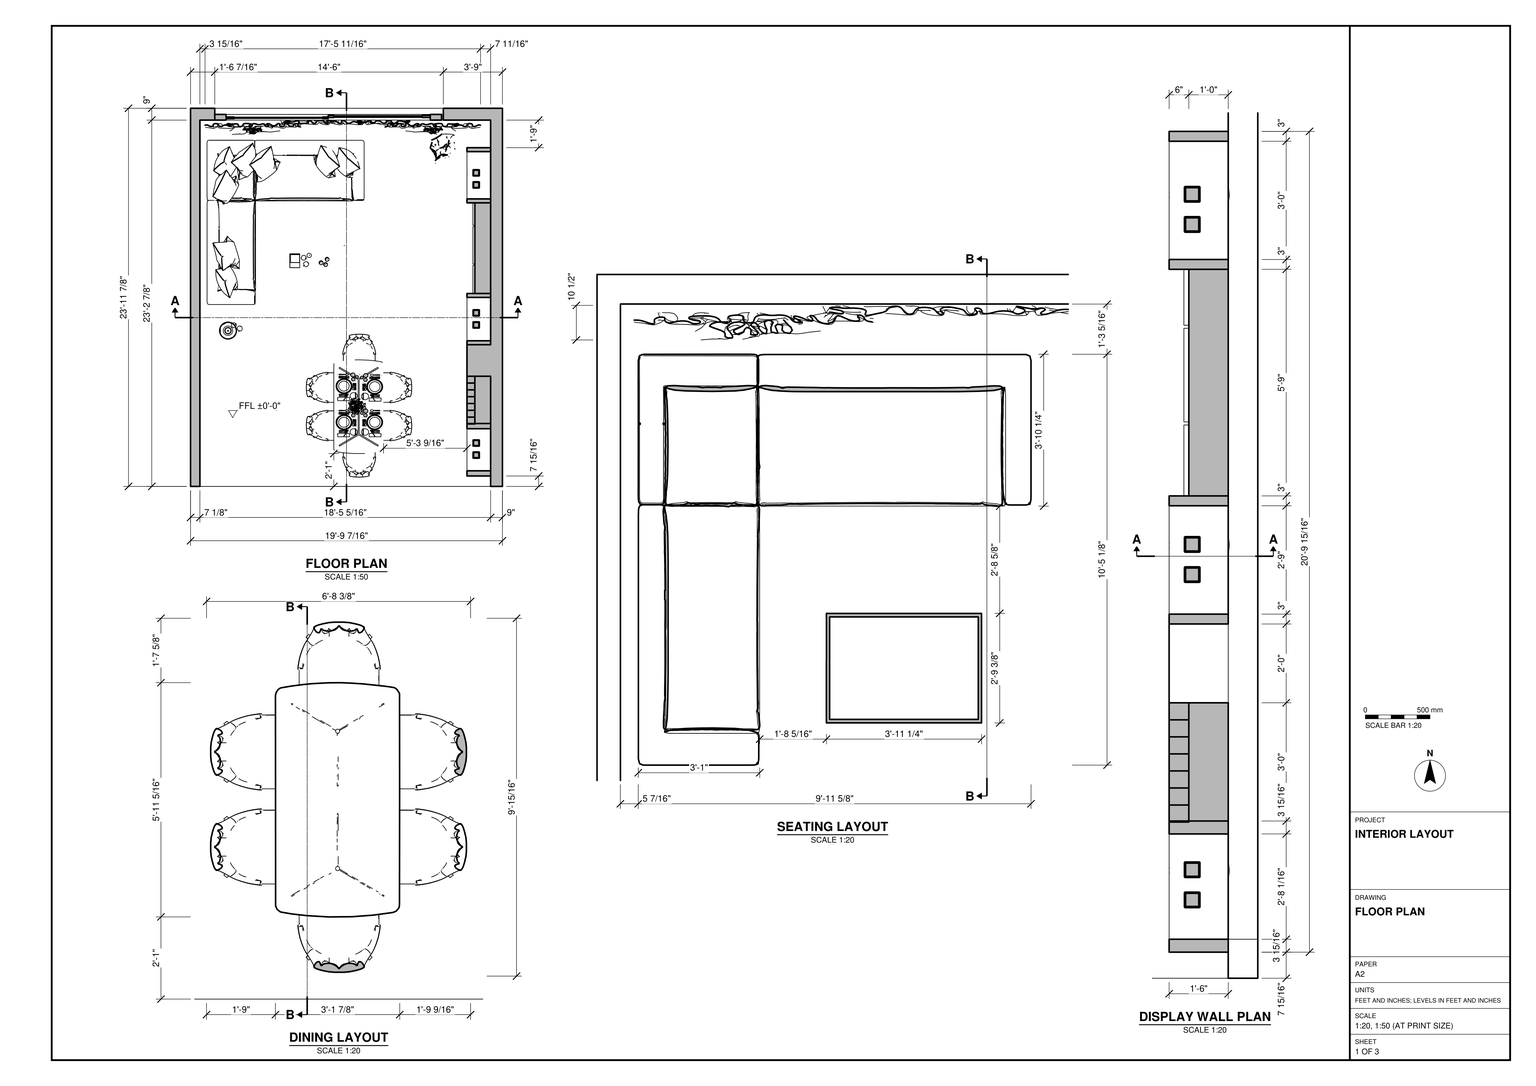
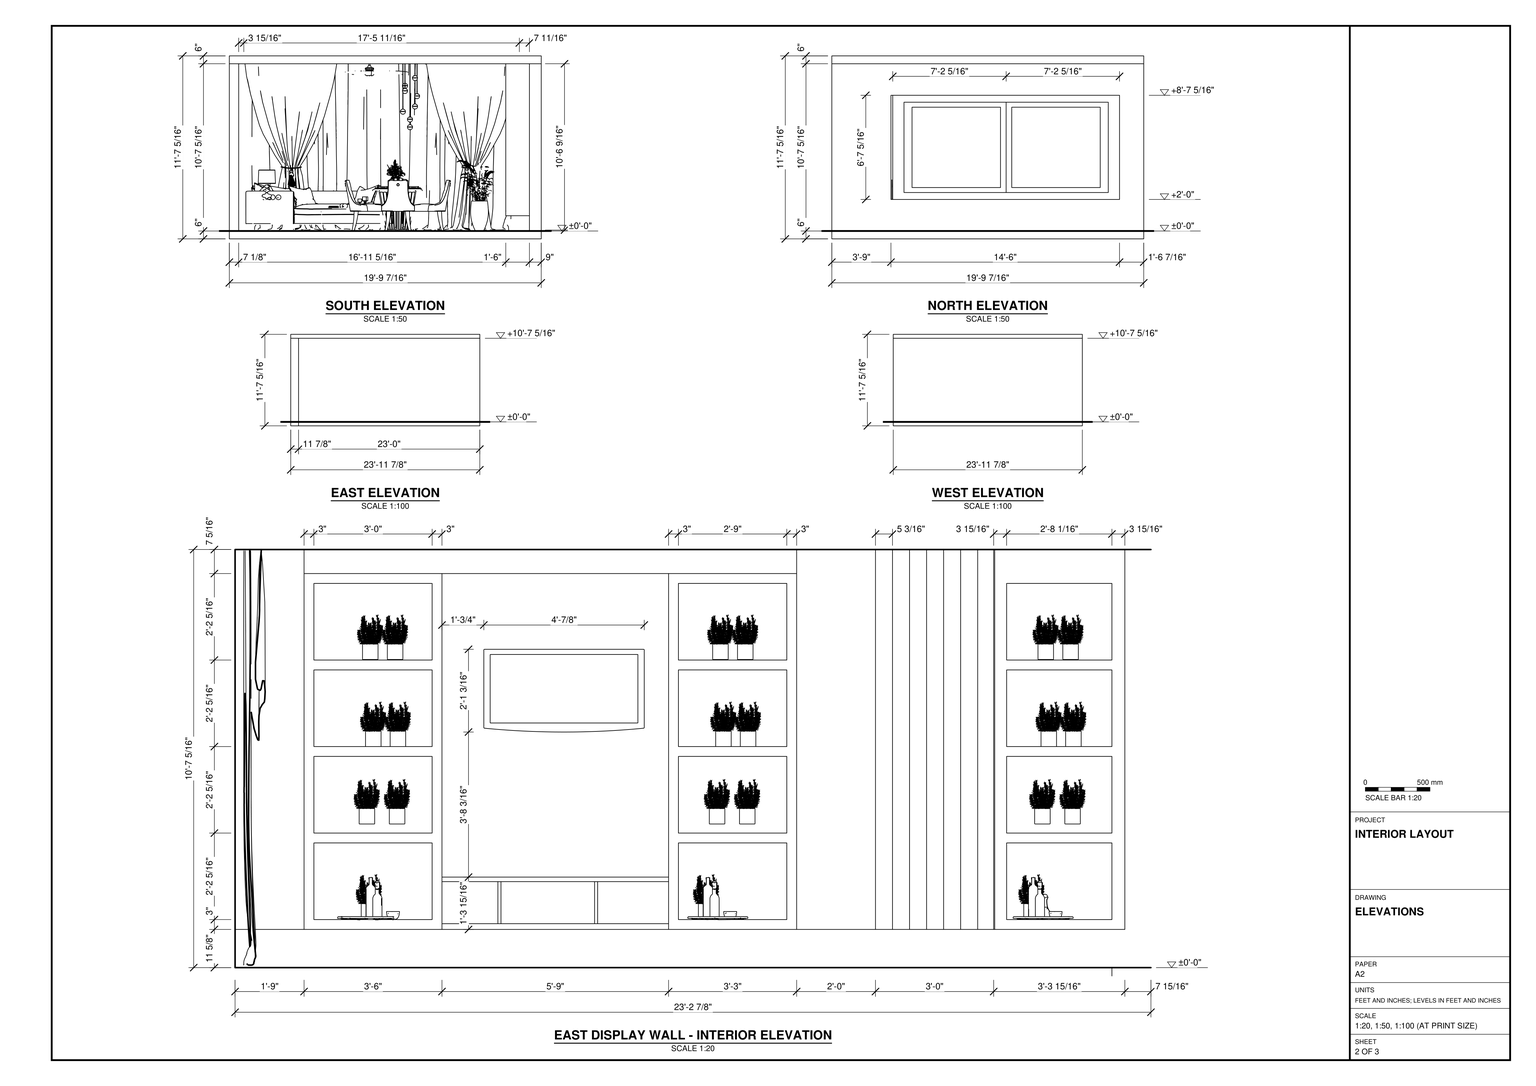
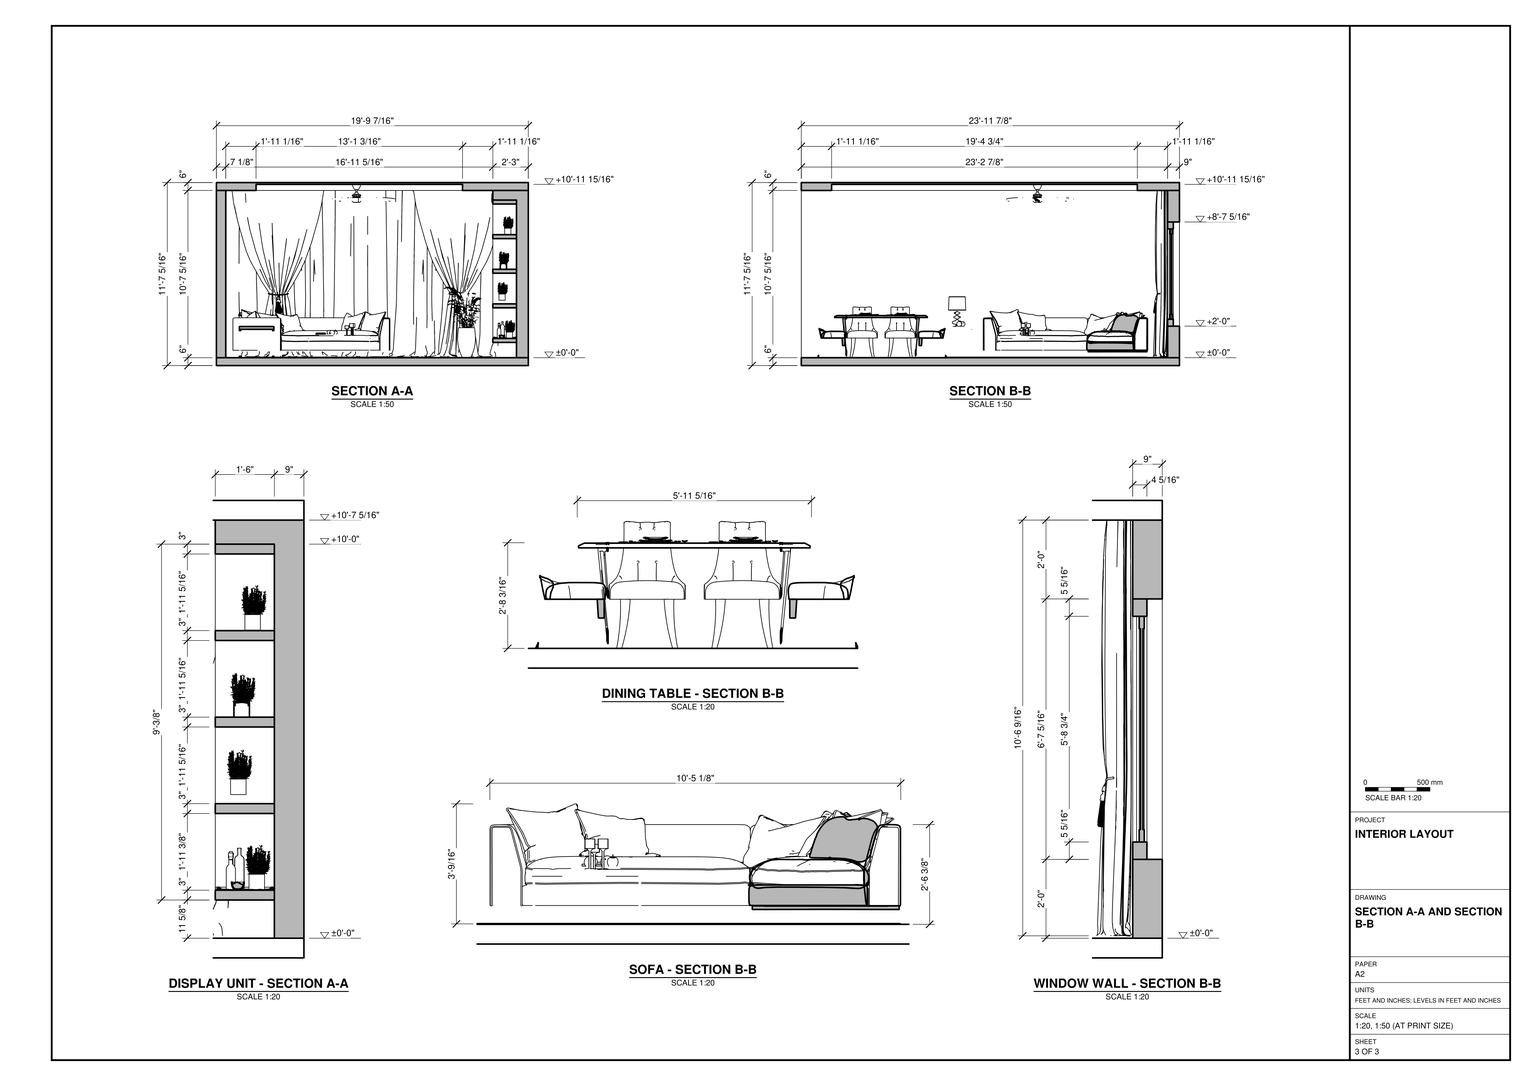
Build the furnished room shown in task_files/diagram_01.pdf. Work in feet and inches. Set the finished floor at ±0'-0" and orient the north window wall as shown in plan. The overall model measures 19'-9 7/16" east to west, 23'-11 7/8" north to south and 11'-7 5/16" high.

Model the floor slab, the west wall at 7 1/8" thick, and the north and east walls at 9" thick. Leave the south side open as drawn. Follow the sections for the slab thicknesses and recessed ceiling. Fit the wide, two-panel window into the north wall, with curtains on the room side. Place the L-shaped sofa in the northwest corner with the coffee table inside the L. In the southern part of the room, orient the dining table lengthwise north to south and arrange the chairs as shown in the dining layout.

Build the east display wall from its plan, interior elevation and section. Match the depth and spacing of the open shelf bays, the screen and low cabinet between the bays, and the vertically divided panel toward the dining end. Include the plants and shelf objects where shown. Decor and loose items may be any suitable library components.

Keep the shell elements and each furniture or joinery piece in separate groups or components, and use components for repeated parts. Save one SketchUp model as output_files/living_and_dining_room_with_built_in_display_shelving.skp.

# SketchUp Ruby script. Lengths in inches.
U = 1.inch
M = Sketchup.active_model
def pt(a) = Geom::Point3d.new(a.map { |v| v * U })
def face(e, loops, mat)
  f = e.add_face(loops[0].map { |a| pt(a) })
  loops[1..].each { |l| e.add_face(l.map { |a| pt(a) }).erase! }
  f.material = f.back_material = mat if mat
  f
end
# faces: each face lists its corners as indices into pts; further lists are holes
def faces(e, pts, list, mat = nil) = list.each { |f| face(e, (f[0].is_a?(Array) ? f : [f]).map { |l| l.map { |i| pts[i] } }, mat) }
# xy, xz, yz: faces in a plane at the given z, y or x. An outline is a flat list of corners, or four numbers for a rectangle; further outlines are holes
def ring(l) = l.size == 4 ? [[l[0], l[1]], [l[2], l[1]], [l[2], l[3]], [l[0], l[3]]] : l.each_slice(2).to_a
def flat(e, list, mat, &to3) = list.each { |f| face(e, (f[0].is_a?(Array) ? f : [f]).map { |l| ring(l).map { |u, v| to3.(u, v) } }, mat) }
def xy(e, z, list, mat = nil) = flat(e, list, mat) { |x, y| [x, y, z] }
def xz(e, y, list, mat = nil) = flat(e, list, mat) { |x, z| [x, y, z] }
def yz(e, x, list, mat = nil) = flat(e, list, mat) { |y, z| [x, y, z] }
def lines(e, pts, list) = list.each { |a, b| e.add_line(pt(pts[a]), pt(pts[b])) }
# prism: a flat outline (further loops are holes) pulled along v
def prism(e, loops, v, mat = nil)
  f = face(e, loops, mat); d = Geom::Vector3d.new(v.map { |x| x * U })
  f.pushpull(f.normal.samedirection?(d) ? d.length : -d.length)
end
def box(e, o, s, mat = nil) = prism(e, [[o, [o[0] + s[0], o[1], o[2]], [o[0] + s[0], o[1] + s[1], o[2]], [o[0], o[1] + s[1], o[2]]]], [0, 0, s[2]], mat)
def at(x, y, z, deg = 0) = Geom::Transformation.translation(pt([x, y, z])) * Geom::Transformation.rotation(ORIGIN, Z_AXIS, deg.degrees)
def axes(o, x, y, z) = Geom::Transformation.new([*x, 0, *y, 0, *z, 0, *pt(o).to_a, 1])
def part(name) = M.definitions.add(name)
# library, detail: a bought-in or finely detailed component or shape, given as its bounding box
def library(name, o, s) = part(name).tap { |d| box(d.entities, o, s) }
def detail(e, o, s) = box(e.add_group.entities, o, s)
def put(e, d, t, mat = nil) = e.add_instance(d, t).tap { |i| i.material = mat if mat }
def group(e, t, mat = nil) = e.add_group.tap { |g| g.transformation = t; g.material = mat if mat }.entities
root = M.entities
M.materials.add("Decor - Oil Bottle - Label").color = [52, 51, 50]
M.materials.add("Decor - Oil Bottles - Black Glass").color = [0, 0, 0]
M.materials["Decor - Oil Bottles - Black Glass"].alpha = 0.45
M.materials.add("[Carrera Marble]").color = [207, 207, 207]
M.materials.add("[Color D02]").color = [255, 241, 201]
M.materials.add("[Stone Brushed Khaki]").color = [226, 197, 133]
M.materials.add("[Translucent_Glass_Safety]").color = [204, 235, 244]
M.materials["[Translucent_Glass_Safety]"].alpha = 0.5
M.materials.add("[Translucent_Glass_Sky_Reflection]").color = [125, 138, 183]
M.materials["[Translucent_Glass_Sky_Reflection]"].alpha = 0.52
M.materials.add("[Wood Veneer 01]").color = [120, 70, 37]
c1 = library("Group14",[-64.97,9.24,0.31],[138.52,9.93,292.57])
c2 = library("Group16",[86.37,-10.76,76.46],[21.79,14.87,35.97])
c3 = library("Group22",[48.82,-10.91,0.23],[97.72,18.57,293.12])
c4 = library("Group24",[44.03,2.01,0.26],[103.73,11,292.35])
c5 = library("Group27",[-106.21,-10.76,76.46],[21.8,14.87,35.97])
c6 = library("Group35",[-145.81,2.01,0.26],[103.73,11,292.35])
c7 = library("Group33",[-144.59,-10.91,0.23],[97.72,18.57,293.12])
c8 = part("rem")
g1 = group(c8.entities,at(-145.81,-10.91,0.23))
put(g1,c1,at(145.81,10.91,-0.23))
put(g1,c2,at(145.81,10.91,-0.23))
put(g1,c3,at(145.81,10.91,-0.23))
put(g1,c4,at(145.81,10.91,-0.23))
put(g1,c5,at(145.81,10.91,-0.23))
put(g1,c6,at(145.81,10.91,-0.23))
put(g1,c7,at(145.81,10.91,-0.23))
c9 = part("Sliding window")
xy(c9.entities,0,[[0,0,4.33,55.51]])
xy(c9.entities,2.76,[[0,2.76,2,27.76],[3.15,2.76,4.33,27.76],[0,27.76,0.82,52.76],[0.82,27.76,2.36,52.76],[2.36,27.76,4.33,52.76]])
xy(c9.entities,4.72,[[2,4.72,2.4,26.38],[2.76,4.72,3.15,26.38],[0.82,29.13,1.22,50.79],[1.97,29.13,2.36,50.79]])
xy(c9.entities,36.61,[[2,4.72,2.4,26.38],[2.76,4.72,3.15,26.38],[0.82,29.13,1.22,50.79],[1.97,29.13,2.36,50.79]])
xy(c9.entities,38.58,[[0,2.76,2,27.76],[3.15,2.76,4.33,27.76],[0,27.76,0.82,52.76],[0.82,27.76,2.36,52.76],[2.36,27.76,4.33,52.76]])
xy(c9.entities,41.34,[[0,0,4.33,55.51]])
xz(c9.entities,0,[[0,0,4.33,41.34]])
xz(c9.entities,2.76,[[0,2.76,2,38.58],[3.15,2.76,4.33,38.58]])
xz(c9.entities,4.72,[[2,4.72,2.4,36.61],[2.76,4.72,3.15,36.61]])
xz(c9.entities,26.38,[[2,4.72,2.4,36.61],[2.76,4.72,3.15,36.61]])
xz(c9.entities,27.76,[[0.82,2.76,2,38.58],[2,2.76,2.36,38.58],[2.36,2.76,3.15,38.58]])
xz(c9.entities,29.13,[[0.82,4.72,1.22,36.61],[1.97,4.72,2.36,36.61]])
xz(c9.entities,50.79,[[0.82,4.72,1.22,36.61],[1.97,4.72,2.36,36.61]])
xz(c9.entities,52.76,[[0,2.76,0.82,38.58],[0.82,2.76,2.36,38.58],[2.36,2.76,4.33,38.58]])
xz(c9.entities,55.51,[[0,0,4.33,41.34]])
yz(c9.entities,0,[[[0,0,55.51,41.34],[2.76,2.76,52.76,38.58]]])
yz(c9.entities,0.82,[[[27.76,2.76,52.76,38.58],[29.13,4.72,50.79,36.61]]])
yz(c9.entities,1.22,[[29.13,4.72,50.79,36.61]],"[Translucent_Glass_Sky_Reflection]")
yz(c9.entities,1.97,[[29.13,4.72,50.79,36.61]],"[Translucent_Glass_Sky_Reflection]")
yz(c9.entities,2,[[[2.76,2.76,27.76,38.58],[4.72,4.72,26.38,36.61]]])
yz(c9.entities,2.36,[[[27.76,2.76,52.76,38.58],[29.13,4.72,50.79,36.61]]])
yz(c9.entities,2.4,[[4.72,4.72,26.38,36.61]],"[Translucent_Glass_Safety]")
yz(c9.entities,2.76,[[4.72,4.72,26.38,36.61]],"[Translucent_Glass_Safety]")
yz(c9.entities,3.15,[[[2.76,2.76,27.76,38.58],[4.72,4.72,26.38,36.61]]])
yz(c9.entities,4.33,[[[0,0,55.51,41.34],[2.76,2.76,52.76,38.58]]])
c10 = library("dinning+table+2",[29.07,47.92,0],[99.06,67.68,49.4])
c11 = library("Cluster pendant light",[0,0,0],[15.54,15.54,54.85])
c12 = library("Untitled",[82.71,28.87,-11.8125],[39.77,1.97,25.2])
c13 = library("Avation+Styled+Ceiling+Fan_JSB",[-19.77,-29.63,-13.8125],[51.59,58.16,13.8125])
c14 = library("Group3\#3",[-238.15,54.18,0],[46.4,43.96,56.68])
c15 = library("迷迭香盆栽   Potted rosemary    盆栽 Potted plants     迷迭香   Rosema",[-0.43,-2,0.01],[7.68,8.25,13.59])
c16 = library("Tepsi",[27.43,-114.7,10.73],[90.81,90.81,4.36])
c17 = library("Utensílios de cozinha - Galheteiro ",[91.875,-459.8125,1.36],[84.84,84.82,188.36])
c18 = part("Group\#1")
xy(c18.entities,115.6875,[[0,0,6,5.1875]])
xz(c18.entities,0,[[0,0,6,115.6875]])
yz(c18.entities,0,[[0,0,5.1875,115.6875]])
c19 = library("Group\#11",[0,0,0],[145.32,155.63,46.53])
c20 = library("Group325\#1",[30.57,-11.72,-14.39],[18.62,18.62,11.32])
c21 = library("Group318\#2",[50.77,-2.74,-14.76],[26.73,29.52,13.62])
c22 = library("Group\#44",[-0.82,-0.34,0],[4.09,3.62,11.67])
c23 = library("olive_Defintion19",[-63.02,-346.37,-115.47],[230.93,1000,230.94])
c24 = part("olive_Defintion")
p = [[49.84,-436.47,-188.95],[50.23,563.53,-187],[87.34,563.53,-190.7],[87.34,-436.47,-192.68],[124.45,563.53,-187],[124.84,-436.47,-188.95],
  [14.53,563.53,-176.21],[13.77,-436.47,-178.05],[160.15,563.53,-176.21],[160.91,-436.47,-178.05],[-19.44,-436.47,-160.25],[-18.34,563.53,-158.6],
  [193.02,563.53,-158.6],[194.12,-436.47,-160.25],[-45.45,563.53,-137.57],[-46.84,-436.47,-139],[220.13,563.53,-137.57],[221.52,-436.47,-139],
  [-65.45,-436.47,-117.73],[-63.87,563.53,-116.52],[238.55,563.53,-116.52],[240.13,-436.47,-117.73],[-77.94,563.53,-95.46],[-79.67,-436.47,-96.45],
  [252.625,563.53,-95.46],[254.35,-436.47,-96.45],[-65.45,-436.47,117.65],[-63.87,563.53,116.4375],[-77.94,563.53,95.375],[-79.67,-436.47,96.37],
  [252.625,563.53,95.375],[238.55,563.53,116.4375],[240.13,-436.47,117.65],[254.35,-436.47,96.37],[-45.45,563.53,137.49],[-46.84,-436.47,138.92],
  [220.13,563.53,137.49],[221.52,-436.47,138.92],[-19.44,-436.47,160.17],[-18.34,563.53,158.52],[193.02,563.53,158.52],[194.12,-436.47,160.17],
  [14.53,563.53,176.13],[13.77,-436.47,177.96],[160.15,563.53,176.13],[160.91,-436.47,177.96],[49.84,-436.47,188.87],[50.23,563.53,186.92],
  [124.45,563.53,186.92],[124.84,-436.47,188.87],[87.34,563.53,190.61],[87.34,-436.47,192.6]]
faces(c24.entities,p,[[0,1,2,3],[2,4,5,3],[6,1,0,7],[5,4,8,9],[10,11,6,7],[8,12,13,9],[14,11,10,15],[13,12,16,17],
  [18,19,14,15],[16,20,21,17],[22,19,18,23],[21,20,24,25],[26,27,28,29],[30,31,32,33],[34,27,26,35],[32,31,36,37],
  [38,39,34,35],[36,40,41,37],[42,39,38,43],[41,40,44,45],[46,47,42,43],[44,48,49,45],[50,47,46,51],[49,48,50,51]],"Decor - Oil Bottle - Label")
c25 = part("Group32\#1")
put(c25.entities,c23,axes([15235.87,28195.44,20659.33],[-10.1187,-7.58183,0],[0,0,12.64406],[-7.58183,10.1187,0]),"Decor - Oil Bottles - Black Glass")
put(c25.entities,c24,axes([15235.87,28195.44,20659.33],[-6.07632,-4.55292,0],[0,0,7.59281],[-4.55292,6.07632,0]),"Decor - Oil Bottle - Label")
c26 = part("Group31\#1")
put(c26.entities,c25,at(0,0,0))
xy(root,-6,[[0,0,237.4375,11.875],[0,11.875,237.4375,287.875]])
xy(root,0,[[0,0,7.125,11.875],[7.125,0,228.4375,278.875],[228.4375,0,237.4375,11.875],[0,11.875,7.125,11.875,7.125,278.875,228.4375,278.875,228.4375,11.875,237.4375,11.875,237.4375,287.875,0,287.875]])
xy(root,11.625,[[210.4375,7.9375,228.4375,11.875],[210.4375,11.875,228.4375,47.875],[216.4375,47.875,228.4375,83.875],[210.4375,78.6875,216.4375,83.875],[210.4375,83.875,228.4375,107.875],
  [210.4375,107.875,228.4375,146.875],[217.6875,146.875,228.4375,215.875],[210.4375,215.875,228.4375,257.875]])
xy(root,13.375,[[214.9375,146.875,216.4375,168.47],[216.4375,146.875,216.4375,198.85,214.9375,198.85,214.9375,215.875,217.6875,215.875,217.6875,146.875],[214.9375,169.41,216.4375,197.91]])
xy(root,14.625,[[210.4375,11.875,228.4375,43.9375],[210.4375,110.875,228.4375,143.875],[210.4375,218.875,228.4375,254.875]],"[Wood Veneer 01]")
xy(root,24,[[18.4375,278.875,192.4375,287.875]])
xy(root,26.1875,[[214.9375,146.875,216.4375,168.47],[216.4375,146.875,217.6875,146.875,217.6875,215.875,214.9375,215.875,214.9375,198.85,216.4375,198.85],[214.9375,169.41,216.4375,197.91]],"[Stone Brushed Khaki]")
xy(root,27.5625,[[216.4375,146.875,217.6875,215.875]])
xy(root,37.97,[[210.4375,11.875,228.4375,43.9375],[210.4375,110.875,228.4375,143.875],[210.4375,218.875,228.4375,254.875]])
xy(root,40.97,[[210.4375,11.875,228.4375,43.9375],[210.4375,110.875,228.4375,143.875],[210.4375,218.875,228.4375,254.875]],"[Wood Veneer 01]")
xy(root,64.3125,[[210.4375,11.875,228.4375,43.9375],[210.4375,110.875,228.4375,143.875],[210.4375,218.875,228.4375,254.875]])
xy(root,67.3125,[[210.4375,11.875,228.4375,43.9375],[210.4375,110.875,228.4375,143.875],[210.4375,218.875,228.4375,254.875]],"[Wood Veneer 01]")
xy(root,90.66,[[210.4375,11.875,228.4375,43.9375],[210.4375,110.875,228.4375,143.875],[210.4375,218.875,228.4375,254.875]])
xy(root,93.66,[[210.4375,11.875,228.4375,43.9375],[210.4375,110.875,228.4375,143.875],[210.4375,218.875,228.4375,254.875]],"[Wood Veneer 01]")
xy(root,103.3125,[[18.4375,278.875,192.4375,287.875]])
xy(root,117,[[210.4375,11.875,228.4375,43.9375],[210.4375,110.875,228.4375,143.875],[210.4375,218.875,228.4375,254.875]])
xy(root,120,[[210.4375,107.875,228.4375,146.875],[210.4375,146.875,216.4375,215.875],[216.4375,146.875,228.4375,215.875],[210.4375,215.875,228.4375,257.875]])
xy(root,127.3125,[[[7.125,0,7.125,278.875,228.4375,278.875,228.4375,257.875,210.4375,257.875,210.4375,83.875,216.4375,83.875,216.4375,47.875,210.4375,47.875,210.4375,7.9375,228.4375,7.9375,228.4375,0],[30.2,23.07,187.37,255.8]],[210.4375,7.9375,210.4375,47.875,216.4375,47.875,216.4375,83.875,228.4375,83.875,228.4375,7.9375]])
xy(root,127.3125,[[0,0,0,287.875,237.4375,287.875,237.4375,0,228.4375,0,228.4375,83.875,210.4375,83.875,210.4375,257.875,228.4375,257.875,228.4375,278.875,7.125,278.875,7.125,0],[210.4375,7.9375,228.4375,47.875],[216.4375,47.875,228.4375,83.875]],"[Wood Veneer 01]")
xy(root,131.9375,[[30.2,23.07,187.37,255.8]])
xy(root,133.3125,[[0,0,237.4375,287.875]])
xz(root,0,[[0,-6,237.4375,0],[0,0,7.125,127.3125],[228.4375,0,237.4375,127.3125],[0,127.3125,237.4375,133.3125]])
xz(root,7.9375,[[210.4375,11.625,228.4375,127.3125]],"[Wood Veneer 01]")
xz(root,11.875,[[210.4375,14.625,228.4375,37.97],[210.4375,40.97,228.4375,64.3125],[210.4375,67.3125,228.4375,90.66],[210.4375,93.66,228.4375,117]],"[Wood Veneer 01]")
xz(root,23.07,[[30.2,127.3125,187.37,131.9375]])
xz(root,43.9375,[[210.4375,14.625,228.4375,37.97],[210.4375,40.97,228.4375,64.3125],[210.4375,67.3125,228.4375,90.66],[210.4375,93.66,228.4375,117]],"[Wood Veneer 01]")
xz(root,47.875,[[210.4375,11.625,216.4375,127.3125],[216.4375,11.625,228.4375,127.3125]])
xz(root,83.875,[[210.4375,11.625,216.4375,127.3125],[216.4375,11.625,228.4375,127.3125]])
xz(root,107.875,[[210.4375,11.625,228.4375,120]])
xz(root,110.875,[[210.4375,14.625,228.4375,37.97],[210.4375,40.97,228.4375,64.3125],[210.4375,67.3125,228.4375,90.66],[210.4375,93.66,228.4375,117]],"[Wood Veneer 01]")
xz(root,143.875,[[210.4375,14.625,228.4375,37.97],[210.4375,40.97,228.4375,64.3125],[210.4375,67.3125,228.4375,90.66],[210.4375,93.66,228.4375,117]],"[Wood Veneer 01]")
xz(root,146.875,[[217.6875,11.625,217.6875,13.375,216.4375,13.375,216.4375,26.1875,217.6875,26.1875,217.6875,27.5625,216.4375,27.5625,216.4375,120,228.4375,120,228.4375,11.625],[214.9375,13.375,216.4375,26.1875]])
xz(root,146.875,[[210.4375,11.625,210.4375,120,216.4375,120,216.4375,27.5625,217.6875,27.5625,217.6875,26.1875,214.9375,26.1875,214.9375,13.375,217.6875,13.375,217.6875,11.625]],"[Wood Veneer 01]")
xz(root,168.47,[[214.9375,13.375,216.4375,26.1875]])
xz(root,169.41,[[214.9375,13.375,216.4375,26.1875]])
xz(root,197.91,[[214.9375,13.375,216.4375,26.1875]])
xz(root,198.85,[[214.9375,13.375,216.4375,26.1875]],"[Stone Brushed Khaki]")
xz(root,215.875,[[217.6875,11.625,228.4375,11.625,228.4375,120,216.4375,120,216.4375,27.5625,217.6875,27.5625,217.6875,26.1875,214.9375,26.1875,214.9375,13.375,217.6875,13.375]])
xz(root,215.875,[[210.4375,11.625,217.6875,11.625,217.6875,13.375,214.9375,13.375,214.9375,26.1875,217.6875,26.1875,217.6875,27.5625,216.4375,27.5625,216.4375,120,210.4375,120]],"[Wood Veneer 01]")
xz(root,218.875,[[210.4375,14.625,228.4375,37.97],[210.4375,40.97,228.4375,64.3125],[210.4375,67.3125,228.4375,90.66],[210.4375,93.66,228.4375,117]])
xz(root,254.875,[[210.4375,14.625,228.4375,37.97],[210.4375,40.97,228.4375,64.3125],[210.4375,67.3125,228.4375,90.66],[210.4375,93.66,228.4375,117]],"[Wood Veneer 01]")
xz(root,255.8,[[30.2,127.3125,187.37,131.9375]])
xz(root,257.875,[[210.4375,120,228.4375,127.3125]])
xz(root,257.875,[[210.4375,11.625,228.4375,120]],"[Wood Veneer 01]")
xz(root,278.875,[[[7.125,0,228.4375,127.3125],[18.4375,24,192.4375,103.3125]]],"[Color D02]")
xz(root,287.875,[[0,-6,237.4375,0],[[0,0,237.4375,127.3125],[18.4375,24,192.4375,103.3125]],[0,127.3125,237.4375,133.3125]])
yz(root,0,[[0,-6,287.875,0],[0,0,287.875,127.3125],[0,127.3125,287.875,133.3125]])
yz(root,7.125,[[0,0,278.875,127.3125]],"[Color D02]")
yz(root,18.4375,[[278.875,24,287.875,103.3125]])
yz(root,30.2,[[23.07,127.3125,255.8,131.9375]])
yz(root,187.37,[[23.07,127.3125,70.95,131.9375],[70.95,127.3125,107.875,131.9375],[107.875,127.3125,255.8,131.9375]])
yz(root,192.4375,[[278.875,24,287.875,103.3125]])
yz(root,210.4375,[[83.875,11.625,107.875,127.3125]],"[Color D02]")
yz(root,210.4375,[[[7.9375,11.625,47.875,127.3125],[11.875,14.625,43.9375,37.97],[11.875,67.3125,43.9375,90.66],[11.875,93.66,43.9375,117],[11.875,40.97,43.9375,64.3125]],[[107.875,11.625,146.875,120],[110.875,93.66,143.875,117],[110.875,67.3125,143.875,90.66],[110.875,14.625,143.875,37.97],[110.875,40.97,143.875,64.3125]],[[215.875,11.625,257.875,120],[218.875,93.66,254.875,117],[218.875,67.3125,254.875,90.66],[218.875,14.625,254.875,37.97],[218.875,40.97,254.875,64.3125]],[107.875,120,257.875,127.3125]],"[Wood Veneer 01]")
yz(root,214.9375,[[146.875,13.375,168.47,26.1875],[169.41,13.375,197.91,26.1875],[198.85,13.375,215.875,26.1875]],"[Stone Brushed Khaki]")
yz(root,216.4375,[[47.875,11.625,78.6875,127.3125],[78.6875,11.625,83.875,127.3125],[146.875,13.375,168.47,26.1875],[169.41,13.375,197.91,26.1875],[197.91,13.375,198.85,26.1875]])
yz(root,216.4375,[[146.875,27.5625,215.875,120]],"[Carrera Marble]")
yz(root,216.4375,[[168.47,13.375,169.41,26.1875]],"[Stone Brushed Khaki]")
yz(root,217.6875,[[146.875,11.625,215.875,13.375]])
yz(root,217.6875,[[146.875,26.1875,215.875,27.5625]],"[Stone Brushed Khaki]")
yz(root,228.4375,[[[7.9375,11.625,47.875,127.3125],[11.875,14.625,43.9375,37.97],[11.875,93.66,43.9375,117],[11.875,67.3125,43.9375,90.66],[11.875,40.97,43.9375,64.3125]],[47.875,11.625,83.875,127.3125],[[107.875,11.625,146.875,120],[110.875,93.66,143.875,117],[110.875,67.3125,143.875,90.66],[110.875,14.625,143.875,37.97],[110.875,40.97,143.875,64.3125]],[146.875,11.625,215.875,120],[[215.875,11.625,257.875,120],[218.875,93.66,254.875,117],[218.875,67.3125,254.875,90.66],[218.875,14.625,254.875,37.97],[218.875,40.97,254.875,64.3125]]])
yz(root,228.4375,[[0,0,0,127.3125,7.9375,127.3125,7.9375,11.625,278.875,11.625,278.875,0],[257.875,11.625,278.875,127.3125]],"[Color D02]")
yz(root,228.4375,[[11.875,14.625,43.9375,37.97],[110.875,14.625,143.875,37.97],[218.875,14.625,254.875,37.97],[11.875,40.97,43.9375,64.3125],[110.875,40.97,143.875,64.3125],
  [218.875,40.97,254.875,64.3125],[11.875,67.3125,43.9375,90.66],[110.875,67.3125,143.875,90.66],[218.875,67.3125,254.875,90.66],[11.875,93.66,43.9375,117],
  [110.875,93.66,143.875,117],[218.875,93.66,254.875,117]],"[Wood Veneer 01]")
yz(root,237.4375,[[0,-6,11.875,0],[11.875,-6,287.875,0],[0,0,11.875,127.3125],[11.875,0,287.875,127.3125],[0,127.3125,287.875,133.3125]])
put(root,c8,axes([115.2,271.76,0.62],[0.71436,0,0],[0,0.35,0],[0,0,0.43188]))
put(root,c9,axes([18.4375,283.21,24],[0,-1,0],[3.11,0,0],[0,0,1.91861]))
put(root,c10,axes([31.14,147.95,0],[0,-1.1,0],[1.188,0,0],[0,0,1.1]))
put(root,c11,at(130.16,87.23,77.09))
put(root,c12,axes([184.5625,304.75,83.55],[0,-1.2285,0],[1,0,0],[0,0,1]))
put(root,c13,at(106.65,179.77,131.9375))
put(root,c14,at(403.03,184.57,0))
put(root,c15,at(220.03,34.3,14.74))
put(root,c16,axes([204.91,46.79,12.49],[0.2016,0,0],[0,0.2016,0],[0,0,0.2016]))
put(root,c17,axes([210.02,47.3,14.6],[0.03941,0.01056,0],[-0.01056,0.03941,0],[0,0,0.0408]))
put(root,c15,at(214.4,30.98,43.73))
put(root,c15,at(215.43,29.05,67.31))
put(root,c15,at(218.76,29.96,93.82))
put(root,c15,at(218.76,22.4,93.82))
put(root,c15,at(215.43,21.55,67.31))
put(root,c15,at(214.4,21.8,43.73))
put(root,c15,at(214.4,120.86,43.73))
put(root,c15,at(218.76,121.46,93.82))
put(root,c15,at(218.76,129.03,93.82))
put(root,c15,at(214.4,130.05,43.73),"[Wood Veneer 01]")
put(root,c16,axes([204.91,145.85,12.49],[0.2016,0,0],[0,0.2016,0],[0,0,0.2016]))
put(root,c15,at(215.43,120.61,67.31))
put(root,c15,at(215.43,128.11,67.31))
put(root,c15,at(214.4,236.67,43.73))
put(root,c15,at(215.43,227.23,67.31))
put(root,c16,axes([204.91,252.48,12.49],[0.2016,0,0],[0,0.2016,0],[0,0,0.2016]))
put(root,c15,at(214.4,227.48,43.73))
put(root,c15,at(218.76,228.09,93.82))
put(root,c15,at(215.43,234.73,67.31))
put(root,c15,at(218.76,235.65,93.82),"[Wood Veneer 01]")
put(root,c15,at(220.03,133.37,14.74))
put(root,c15,at(220.03,236.04,14.74))
put(root,c11,at(130.16,65.98,77.09))
put(root,c18,at(210.4375,78.6875,11.625),"[Wood Veneer 01]")
put(root,c18,at(210.4375,73.5,11.625),"[Wood Veneer 01]")
put(root,c18,at(210.4375,68.3125,11.625),"[Wood Veneer 01]")
put(root,c18,at(210.4375,63.125,11.625),"[Wood Veneer 01]")
put(root,c18,at(210.4375,57.9375,11.625),"[Wood Veneer 01]")
put(root,c18,at(210.4375,52.75,11.625),"[Wood Veneer 01]")
put(root,c18,at(210.4375,47.5625,11.625),"[Wood Veneer 01]")
put(root,c19,at(12.55,107.94,-0.06))
put(root,c20,axes([217.0625,37.52,17.74],[-0.0063,-0.21216,0],[-0.21216,0.0063,0],[0,0,0.21226]))
put(root,c21,axes([223.86,38.57,16.82],[-0.0044,-0.14827,0],[-0.14827,0.0044,0],[0,0,0.14834]))
put(root,c22,at(214.67,31.88,14.73,30))
put(root,c26,axes([218.94,67.57,-1.81],[-0.00091,-0.00044,0],[0.00044,-0.00091,0],[0,0,0.00101]))
put(root,c22,at(214.67,130.96,14.73,30))
put(root,c26,axes([218.94,166.64,-1.81],[-0.00091,-0.00044,0],[0.00044,-0.00091,0],[0,0,0.00101]))
put(root,c20,axes([217.0625,136.59,17.74],[-0.0063,-0.21216,0],[-0.21216,0.0063,0],[0,0,0.21226]))
put(root,c26,axes([218.94,269.3125,-1.81],[-0.00091,-0.00044,0],[0.00044,-0.00091,0],[0,0,0.00101]))
put(root,c22,at(214.67,233.63,14.73,30))
put(root,c20,axes([217.0625,239.26,17.74],[-0.0063,-0.21216,0],[-0.21216,0.0063,0],[0,0,0.21226]))
